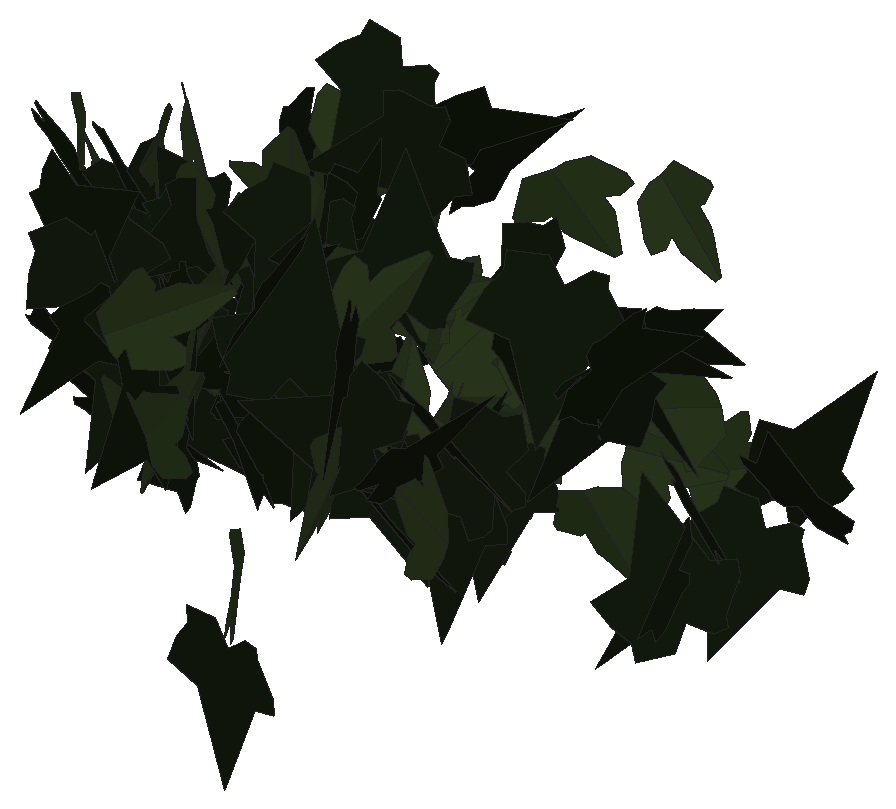
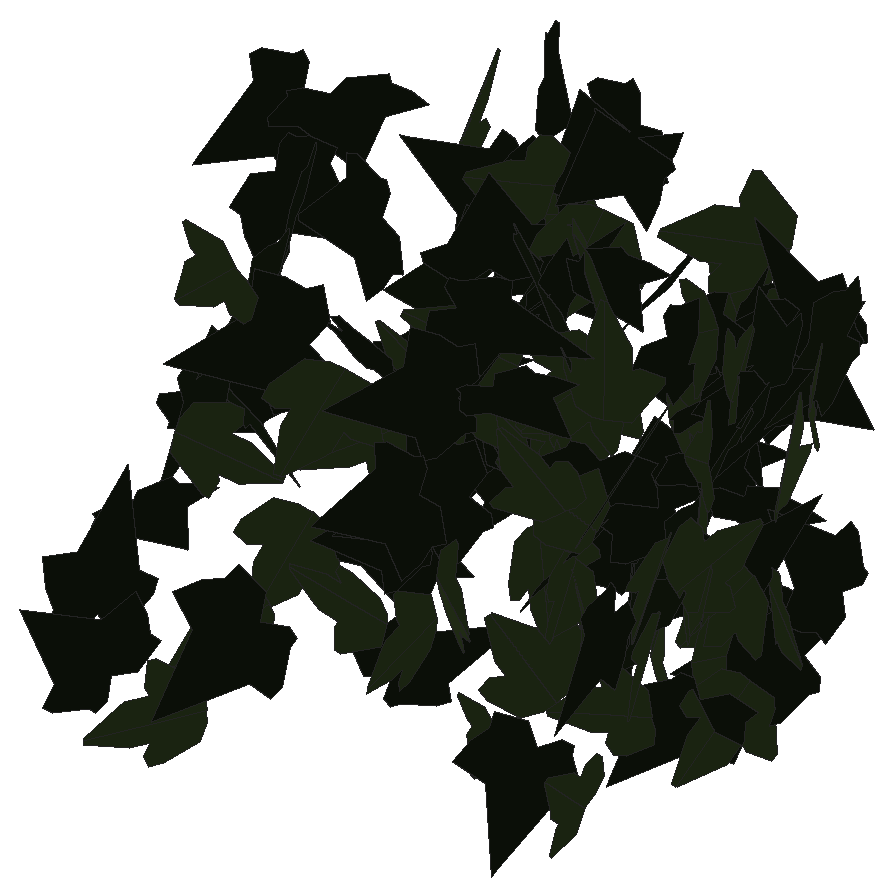
# SketchUp Ruby script. Lengths in inches.
U = 1.inch
M = Sketchup.active_model
def pt(a) = Geom::Point3d.new(a.map { |v| v * U })
def face(e, loops, mat)
  f = e.add_face(loops[0].map { |a| pt(a) })
  loops[1..].each { |l| e.add_face(l.map { |a| pt(a) }).erase! }
  f.material = f.back_material = mat if mat
  f
end
# faces: each face lists its corners as indices into pts; further lists are holes
def faces(e, pts, list, mat = nil) = list.each { |f| face(e, (f[0].is_a?(Array) ? f : [f]).map { |l| l.map { |i| pts[i] } }, mat) }
# xy, xz, yz: faces in a plane at the given z, y or x. An outline is a flat list of corners, or four numbers for a rectangle; further outlines are holes
def ring(l) = l.size == 4 ? [[l[0], l[1]], [l[2], l[1]], [l[2], l[3]], [l[0], l[3]]] : l.each_slice(2).to_a
def flat(e, list, mat, &to3) = list.each { |f| face(e, (f[0].is_a?(Array) ? f : [f]).map { |l| ring(l).map { |u, v| to3.(u, v) } }, mat) }
def xy(e, z, list, mat = nil) = flat(e, list, mat) { |x, y| [x, y, z] }
def xz(e, y, list, mat = nil) = flat(e, list, mat) { |x, z| [x, y, z] }
def yz(e, x, list, mat = nil) = flat(e, list, mat) { |y, z| [x, y, z] }
def lines(e, pts, list) = list.each { |a, b| e.add_line(pt(pts[a]), pt(pts[b])) }
# prism: a flat outline (further loops are holes) pulled along v
def prism(e, loops, v, mat = nil)
  f = face(e, loops, mat); d = Geom::Vector3d.new(v.map { |x| x * U })
  f.pushpull(f.normal.samedirection?(d) ? d.length : -d.length)
end
def box(e, o, s, mat = nil) = prism(e, [[o, [o[0] + s[0], o[1], o[2]], [o[0] + s[0], o[1] + s[1], o[2]], [o[0], o[1] + s[1], o[2]]]], [0, 0, s[2]], mat)
def at(x, y, z, deg = 0) = Geom::Transformation.translation(pt([x, y, z])) * Geom::Transformation.rotation(ORIGIN, Z_AXIS, deg.degrees)
def axes(o, x, y, z) = Geom::Transformation.new([*x, 0, *y, 0, *z, 0, *pt(o).to_a, 1])
def part(name) = M.definitions.add(name)
# library, detail: a bought-in or finely detailed component or shape, given as its bounding box
def library(name, o, s) = part(name).tap { |d| box(d.entities, o, s) }
def detail(e, o, s) = box(e.add_group.entities, o, s)
def put(e, d, t, mat = nil) = e.add_instance(d, t).tap { |i| i.material = mat if mat }
def group(e, t, mat = nil) = e.add_group.tap { |g| g.transformation = t; g.material = mat if mat }.entities
root = M.entities
M.materials.add("efeu1").color = [18, 25, 13]
M.materials.add("efeu2").color = [43, 57, 29]
c1 = part("ivyleaf_10")
p = [[0,0.5,-0.03],[-0.0625,2.02,-0.43],[-0.19,2.01,-0.46],[-0.54,1.05,-0.29],[-0.52,0.625,-0.18],[-0.83,0.76,-0.28],
  [-1.16,0.64,-0.33],[-1.15,0.33,-0.24],[-0.77,-0.39,0.02],[-0.3,-0.51,0.16],[0.04,-0.48,0.23],[-0.02,2.01,-0.4375],
  [-0.06,2.01,-0.43],[0.04,-0.49,0.23],[0.67,-0.49,0.14],[1.38,0.36,-0.2],[1.375,0.51,-0.24],[0.81,0.65,-0.19],
  [0.62,0.59,-0.15],[0.6,1.09,-0.28],[0.5,1.23,-0.31]]
faces(c1.entities,p,[[0,1,2,3,4,5,6,7,8,9,10],[11,12,0,13,14,15,16,17,18,19,20]],"efeu2")
c2 = part("ivyleaf_9")
p = [[1.54,2.16,1.25],[1.36,2.04,1.19],[-0.21,0.99,0.68],[-0.71,1.11,0.82],[-0.85,0.86,0.67],[-0.8,0.17,0.21],
  [-0.9,-0.01,0.1],[-0.67,-0.16,-0.02],[-0.08,-0.08,-0.05],[-0.03,-0.6,-0.4],[0.65,-0.88,-0.66],[0.83,-0.6,-0.49],
  [1.29,-0.42,-0.43],[1.8125,-0.07,-0.26],[1.21,0.44,0.15]]
faces(c2.entities,p,[[0,1,2,3,4,5,6,7,8,9,10,11,12,13,14]],"efeu1")
put(root,c1,axes([545.16,132.69,171.34],[0.0468,-0.12777,0.80813],[0.64002,-0.49853,-0.11589],[0.50968,0.63775,0.07132]))
put(root,c2,axes([545.81,137.93,168.91],[0.10586,0.00489,-0.89003],[-0.6226,0.64092,-0.07053],[0.63604,0.62656,0.07909]))
put(root,c1,axes([545.47,133.17,169.69],[-0.56596,0.35181,0.69168],[0.48132,-0.51238,0.65445],[0.60871,0.73226,0.12562]))
put(root,c2,axes([545.18,131.93,167.14],[0.64135,0.09368,-0.50962],[0.50203,0.08838,0.64805],[0.12825,-0.81439,0.01171]))
put(root,c1,axes([546.17,135.08,168.43],[-0.26299,-0.24108,-0.73681],[-0.41993,-0.60973,0.34938],[-0.65167,0.4902,0.07221]))
put(root,c1,axes([546.54,132.27,166.55],[-0.20531,0.1267,0.79196],[-0.75894,0.23367,-0.23413],[-0.25936,-0.78406,0.0582]))
put(root,c1,axes([546.12,136.41,167.81],[-0.37564,0.62219,0.36467],[-0.21105,0.29833,-0.72641],[-0.68961,-0.43022,0.02367]))
put(root,c2,axes([545.58,131.3,172.08],[0.90183,-0.44317,-0.15553],[-0.13097,0.08607,-1.00465],[0.45103,0.91108,0.01925]))
put(root,c1,axes([546.14,133.78,165.17],[-0.40054,-0.55747,-0.63228],[0.33936,0.53415,-0.68593],[0.77161,-0.5243,-0.02654]))
put(root,c2,axes([545.66,132.53,165.8],[0.77933,-0.17074,0.48973],[0.48275,-0.0843,-0.79762],[0.18957,0.91656,0.01787]))
put(root,c1,axes([545.93,134.91,170.88],[0.18655,-0.26248,0.75231],[0.70853,-0.2988,-0.27994],[0.36448,0.71518,0.15914]))
put(root,c1,axes([546.42,139.27,167.89],[-0.33228,-0.69013,0.41546],[0.17481,0.37693,0.76594],[-0.78634,0.37542,-0.00528]))
put(root,c2,axes([546.96,133.66,166.93],[0.00388,0.08176,1.01596],[-0.82421,-0.59744,0.05123],[0.59962,-0.82174,0.06384]))
put(root,c1,axes([546.66,137.79,164.59],[0.03621,0.51412,-0.64767],[0.0814,0.64293,0.5149],[0.82291,-0.08622,-0.02243]))
put(root,c1,axes([546.3125,133.61,167.44],[-0.74533,0.07894,-0.51976],[0.5144,-0.07659,-0.74928],[-0.10849,-0.90542,0.01806]))
put(root,c1,axes([546.33,134.86,167.47],[-0.43425,0.20169,0.66637],[0.57812,-0.33315,0.47759],[0.38794,0.72224,0.0342]))
put(root,c1,axes([546.875,135.22,168.66],[-0.27817,0.77347,0.24377],[-0.0926,0.22573,-0.8219],[-0.80567,-0.29299,0.0103]))
put(root,c2,axes([546.48,134.53,165.37],[-0.05567,-0.38101,-0.81682],[0.26644,0.77484,-0.37959],[0.86103,-0.2644,0.06465]))
put(root,c2,axes([546.69,132.27,171.05],[0.01681,-0.66358,-0.6588],[-0.00182,0.65889,-0.66371],[0.93507,0.01322,0.01055]))
put(root,c1,axes([546.8,133.1,171.4],[0.05216,-0.14231,-0.80456],[0.16397,-0.78798,0.15001],[-0.80043,-0.1707,-0.0217]))
put(root,c1,axes([546.83,133.8125,165.81],[0.1364,-0.29183,0.87678],[0.4245,-0.76744,-0.32148],[0.82079,0.44541,0.02056]))
put(root,c2,axes([546.61,135.62,167.42],[0.19867,-0.5933,0.60102],[0.2685,-0.54102,-0.62282],[0.80071,0.32862,0.05972]))
put(root,c2,axes([546.55,132.28,171.2],[0.66923,-0.24845,-0.60284],[0.56033,-0.22261,0.71378],[-0.33343,-0.87277,-0.01045]))
put(root,c1,axes([546.86,136.01,165.64],[0.1082,0.05044,0.83793],[0.73557,0.40139,-0.11914],[-0.40448,0.74344,0.00748]))
put(root,c2,axes([547.05,129.99,170.95],[-0.13394,0.09954,0.9014],[0.64776,-0.62719,0.16551],[0.63469,0.66112,0.0213]))
put(root,c2,axes([547.73,131.45,167.94],[-0.72157,-0.40686,-0.14062],[0.12421,0.066,-0.82836],[0.41216,-0.73217,0.00347]))
put(root,c1,axes([547.4,133.38,167.24],[-0.54542,0.41996,0.55461],[0.4431,-0.33359,0.68835],[0.53631,0.70271,-0.00468]))
put(root,c2,axes([547.25,132.66,169.78],[0.13773,-0.58989,0.63667],[0.16032,-0.61626,-0.60565],[0.85301,0.21107,0.01103]))
put(root,c2,axes([547.85,137.7,165.22],[0.50874,0.6559,-0.09298],[-0.06824,-0.06472,-0.82995],[-0.65893,0.5131,0.01417]))
put(root,c2,axes([547.63,133.04,167.75],[0.7859,-0.2609,-0.21098],[-0.19994,0.06735,-0.82808],[0.26945,0.81094,0.0009]))
put(root,c2,axes([548.26,129.63,169.88],[-0.1336,0.27227,-0.80449],[0.18616,-0.78519,-0.29666],[-0.82866,-0.22029,0.06306]))
put(root,c2,axes([548.13,132.27,170.29],[-0.31648,-0.66548,0.32812],[-0.11479,-0.30851,-0.73643],[0.73304,-0.33562,0.02634]))
put(root,c2,axes([547.8125,129.76,171.14],[-0.14827,-0.74749,-0.57441],[0.21913,0.53822,-0.75695],[0.91688,-0.24951,0.08802]))
put(root,c2,axes([548.05,132.17,165.77],[-0.07961,-0.30213,0.75968],[-0.09596,-0.75454,-0.31014],[0.8119,-0.1188,0.03783]))
put(root,c2,axes([548.39,131.83,168.8],[-0.48632,-0.72464,-0.09334],[0.05059,0.07845,-0.8727],[0.72887,-0.48894,-0.0017]))
put(root,c1,axes([548.1,136.88,170.27],[0.66083,0.15914,-0.47947],[0.46747,0.10672,0.67971],[0.19156,-0.80945,-0.00465]))
put(root,c2,axes([549.04,133.41,165.19],[0.13334,-0.42054,0.73686],[-0.07845,0.7366,0.43459],[-0.84479,-0.13478,0.07595]))
put(root,c2,axes([549.04,132.07,171.22],[-0.05277,-0.10494,-0.85907],[0.07109,-0.85828,0.10048],[-0.86253,-0.06432,0.06084]))
put(root,c2,axes([548.43,131.22,169.7],[-0.45887,-0.06523,-0.85105],[0.83339,0.17448,-0.46272],[0.18438,-0.951,-0.02653]))
put(root,c1,axes([548.46,131.86,171.5],[-0.37592,0.35119,-0.72693],[0.53616,-0.49089,-0.51442],[-0.60357,-0.6548,-0.00422]))
put(root,c1,axes([548.8,139.1,168.99],[0.47252,-0.57439,0.48351],[0.30055,-0.37881,-0.74374],[0.68802,0.55996,-0.00717]))
put(root,c2,axes([549.29,134.09,168.18],[0.09813,-0.90153,0.2624],[-0.01305,0.26249,0.90673],[-0.93885,-0.09788,0.01482]))
put(root,c1,axes([549.17,133.9,170.77],[-0.85642,-0.13948,0.0913],[0.09084,0.01019,0.86769],[-0.13977,0.86121,0.00452]))
put(root,c2,axes([549.33,136.95,172.19],[-0.63275,-0.55748,0.05586],[-0.03963,-0.03952,-0.84329],[0.55887,-0.63398,0.00344]))
put(root,c1,axes([549.23,131.6,169.74],[0.28382,-0.62548,0.57367],[0.26298,-0.51032,-0.68651],[0.80695,0.38631,0.02196]))
put(root,c1,axes([549.65,130.17,168.34],[0.19399,-0.80251,0.49862],[0.11645,-0.48483,-0.82562],[0.93759,0.22626,-0.00062]))
put(root,c2,axes([549.18,132.03,167.55],[0.22559,0.04435,0.93346],[0.85859,0.3693,-0.22504],[-0.36897,0.88648,0.04705]))
put(root,c2,axes([549.42,133.8,169.15],[-0.25371,-0.54509,-0.63173],[0.32089,0.54577,-0.59979],[0.77022,-0.40693,0.04179]))
put(root,c1,axes([550.23,133.3125,165.36],[0.37328,-0.29831,0.723],[-0.58107,0.43047,0.47761],[-0.52353,-0.69048,-0.0146]))
put(root,c1,axes([549.53,136.74,164.51],[0.6512,-0.03728,0.52916],[0.52602,-0.06297,-0.65177],[0.0686,0.83673,-0.02548]))
put(root,c1,axes([550.09,133.74,166.36],[-0.01477,-0.60436,-0.67066],[0.0078,0.67064,-0.60452],[0.90276,-0.01568,-0.00575]))
put(root,c2,axes([549.74,131.86,166.56],[0.14508,-0.47662,0.66592],[0.23324,-0.62423,-0.49759],[0.78499,0.27356,0.02478]))
put(root,c1,axes([549.82,131.52,164.05],[0.11579,-0.11647,0.92285],[0.69576,-0.60639,-0.16383],[0.61736,0.70524,0.01155]))
put(root,c1,axes([549.88,133.43,170.73],[-0.79224,0.07311,-0.67145],[0.6691,-0.05628,-0.79559],[-0.09217,-1.03697,-0.00415]))
put(root,c1,axes([549.74,134.01,168.02],[-0.34919,-0.15127,0.8439],[0.79527,0.28326,0.37984],[-0.32029,0.86825,0.0231]))
put(root,c2,axes([550.41,138.07,169.97],[-0.1339,0.58279,-0.65196],[-0.19338,0.6235,0.59706],[0.85282,0.23288,0.03302]))
put(root,c2,axes([550.26,128.59,169.34],[0.19336,-0.32379,-0.95206],[0.64646,-0.70261,0.37024],[-0.7703,-0.67093,0.07174]))
put(root,c2,axes([550.27,133.86,166.68],[0.02412,-0.82645,0.28701],[0.02709,-0.28627,-0.82662],[0.87445,0.03167,0.01769]))
put(root,c1,axes([550.68,133.9,166.92],[-0.13182,-0.91856,-0.06434],[0.01188,0.06329,-0.92796],[0.92073,-0.13232,0.00277]))
put(root,c1,axes([550.25,127.875,170.97],[-0.08395,-0.32421,0.94485],[0.37171,0.86995,0.33153],[-0.92719,0.37812,0.04736]))
put(root,c2,axes([550.1875,131.99,166.06],[0.01643,-0.08115,0.8107],[0.74082,-0.33604,-0.04865],[0.33914,0.73796,0.067]))
put(root,c1,axes([550.85,131.94,169.36],[-0.36836,-0.58269,-0.4797],[0.30729,0.37175,-0.68754],[0.68936,-0.47708,0.05015]))
put(root,c1,axes([550.65,127.78,168.83],[-0.76693,-0.06032,0.58543],[0.5859,0.01263,0.76884],[-0.05562,0.96475,0.02654]))
put(root,c2,axes([551.68,135.07,172.21],[-0.17002,-0.2,-0.85981],[-0.51169,-0.69118,0.26195],[-0.71934,0.53893,0.01688]))
put(root,c2,axes([550.61,136.68,171.42],[0.47077,0.18764,0.67897],[0.6068,0.30675,-0.50551],[-0.35778,0.76716,0.03606]))
put(root,c2,axes([551.21,132.02,172.03],[-0.68965,-0.57396,-0.11611],[0.0952,0.06711,-0.89719],[0.57779,-0.69613,0.00925]))
put(root,c2,axes([551.8,132.42,171.47],[-0.22942,0.59231,0.8468],[-0.32445,0.78226,-0.63507],[-0.98113,-0.39719,0.012]))
put(root,c1,axes([550.73,132.86,169.37],[0.66572,0.15294,0.54034],[0.51472,0.1689,-0.68197],[-0.22454,0.84061,0.03871]))
put(root,c1,axes([551.28,131.89,172.11],[0.70973,-0.65256,-0.03151],[-0.02183,0.02281,-0.96413],[0.65295,0.71007,0.00202]))
put(root,c1,axes([550.9,132.36,168.94],[0.25032,0.20234,-0.90415],[0.69152,0.58252,0.32181],[0.61663,-0.73541,0.00614]))
put(root,c2,axes([551.69,132.625,171.15],[-0.1147,-0.20503,0.845],[-0.38448,-0.75251,-0.23477],[0.77989,-0.40114,0.00853]))
put(root,c2,axes([551.3,135.51,168.51],[0.70923,0.1518,0.48928],[0.47792,0.10484,-0.72529],[-0.18448,0.85523,0.00207]))
put(root,c1,axes([552.17,135.73,165.42],[-0.01734,0.16119,0.86373],[-0.26542,0.82258,-0.15884],[-0.83759,-0.264,0.03245]))
put(root,c2,axes([551.85,133.63,170.91],[0.34291,-0.85103,-0.29467],[-0.07748,0.28626,-0.91691],[0.89726,0.34997,0.03343]))
put(root,c2,axes([552.79,135.65,164.25],[-0.14715,-0.04072,0.84102],[-0.80343,-0.24865,-0.15261],[0.25192,-0.81678,0.00453]))
put(root,c1,axes([552.24,130.46,171.59],[-0.50314,-0.67439,-0.51289],[0.30219,0.41444,-0.84138],[0.79155,-0.58689,-0.0048]))
put(root,c2,axes([552.17,135.83,167.64],[0.68307,-0.26172,0.43688],[0.40721,-0.15828,-0.73149],[0.30586,0.79523,-0.0018]))
put(root,c2,axes([553.19,127.96,172.4375],[-0.32042,0.46666,-0.8797],[-0.4941,0.72783,0.56607],[0.86459,0.58889,-0.00252]))
put(root,c1,axes([552.45,133.1,170.15],[-0.27836,-0.18189,0.85888],[0.69605,0.50339,0.3322],[-0.53504,0.7495,-0.01467]))
put(root,c1,axes([553.07,137.26,170.94],[-0.72191,-0.43332,-0.42296],[0.37441,0.19783,-0.84172],[0.4759,-0.81296,0.02062]))
put(root,c1,axes([553.18,132.19,167.78],[0.9478,-0.12497,0.0511],[-0.04734,0.03178,0.95567],[-0.12644,-0.94864,0.02528]))
put(root,c1,axes([553.47,133.47,168.18],[0.40855,-0.74823,-0.27185],[-0.10636,0.25151,-0.85211],[0.78895,0.42137,0.0259]))
put(root,c1,axes([553.2,133.62,169.74],[-0.00746,-0.2389,-0.91823],[0.38449,0.83872,-0.22134],[0.8674,-0.37384,0.09021]))
put(root,c1,axes([552.75,136.65,166.01],[0.20567,-0.11772,-0.82357],[0.81726,-0.1301,0.22269],[-0.15561,-0.83884,0.08104]))
put(root,c2,axes([553.1875,139.37,166.82],[0.63727,0.57336,0.31985],[0.2324,0.21988,-0.85721],[-0.61403,0.67829,0.00751]))
put(root,c2,axes([553.67,131.71,171.01],[-0.7418,-0.40603,0.51882],[0.46449,0.23175,0.84549],[-0.46721,0.87506,0.01682]))
put(root,c1,axes([553.57,133.47,168.17],[-0.16153,-0.45799,-0.75211],[0.27817,0.69897,-0.48537],[0.83549,-0.32126,0.01619]))
put(root,c2,axes([553.64,134.74,166.32],[-0.628,-0.55094,-0.35137],[0.25787,0.23883,-0.83537],[0.60042,-0.67882,-0.00874]))
put(root,c2,axes([553.8125,128.14,171.21],[-0.70632,-0.31356,0.62057],[0.56165,0.26414,0.77272],[-0.40985,0.90234,-0.01055]))
put(root,c2,axes([553.51,131.49,167.67],[-0.16171,-0.63797,-0.51265],[0.13331,0.49505,-0.65811],[0.80749,-0.20949,0.00598]))
put(root,c2,axes([553.89,129.99,170.19],[-0.60527,-0.76493,0.00311],[-0.00158,-0.00272,-0.97543],[0.76493,-0.60527,0.00045]))
put(root,c2,axes([553.17,131.375,166.61],[0.52185,-0.47308,0.56669],[0.44806,-0.34856,-0.70359],[0.58668,0.68701,0.03326]))
put(root,c2,axes([554.53,134.86,170.52],[-0.87131,0.21897,0.14719],[-0.14336,0.03346,-0.8984],[-0.2215,-0.88302,0.00245]))
put(root,c1,axes([553.5,133.42,169.1],[0.7129,-0.10552,-0.53238],[0.54202,0.09334,0.70731],[-0.02784,-0.88484,0.1381]))
put(root,c2,axes([553.65,131.21,168.91],[0.17319,-0.53157,0.6471],[0.22488,-0.607,-0.55881],[0.80668,0.28334,0.01686]))
put(root,c1,axes([553.76,134.92,168.78],[0.35573,0.29059,0.78873],[0.63634,0.46647,-0.45887],[-0.54918,0.72873,-0.02079]))
put(root,c1,axes([554.14,129.68,171.65],[0.15937,0.34549,-0.88816],[0.38759,0.79915,0.38041],[0.87061,-0.41902,-0.00678]))
put(root,c2,axes([554.94,132.04,168.21],[-0.2914,0.81658,0.2578],[-0.09475,0.2399,-0.86698],[-0.85105,-0.30631,0.00825]))
put(root,c2,axes([555.62,128.2,170.2],[-0.19864,0.01983,0.8844],[-0.84493,-0.27271,-0.18366],[0.262,-0.86443,0.07823]))
put(root,c2,axes([554.96,131.7,167.45],[-0.72751,-0.27777,-0.57547],[0.52874,0.22803,-0.77848],[0.35884,-0.89913,-0.01965]))
put(root,c1,axes([554.83,137.5625,165.63],[0.08556,0.35048,0.7985],[0.18576,0.7766,-0.36077],[-0.85202,0.20451,0.00153]))
put(root,c1,axes([554.83,139.56,164.39],[0.01669,0.07725,0.92151],[0.33051,0.86028,-0.0781],[-0.86366,0.33071,-0.01208]))
put(root,c2,axes([555.76,131.95,168.07],[-0.48516,-0.24244,0.72749],[-0.65445,-0.31773,-0.54234],[0.39963,-0.81466,-0.00498]))
put(root,c2,axes([555.0625,124.6875,167.12],[0.104,-0.92787,0.30072],[0.05473,-0.29639,-0.93345],[0.97384,0.11575,0.02035]))
put(root,c1,axes([555.19,127.73,169.78],[0.1796,-0.37409,0.90819],[0.4549,-0.78658,-0.41396],[0.87053,0.48821,0.02895]))
put(root,c2,axes([554.94,130.53,169.7],[0.68924,-0.47271,0.40824],[0.33898,-0.22753,-0.83576],[0.52461,0.76808,0.00367]))
put(root,c2,axes([555.4,127.9,172.6875],[-0.24287,0.12383,-0.9645],[0.85338,-0.44946,-0.27259],[-0.46619,-0.88726,0.00348]))
put(root,c1,axes([555.7,134.95,165.96],[-0.8588,-0.09893,-0.32733],[0.32491,0.03983,-0.86448],[0.10662,-0.9182,-0.00224]))
put(root,c1,axes([557.08,136.18,168.03],[0.25255,0.01161,-0.84553],[-0.84558,0.01163,-0.25241],[0.00783,0.88237,0.01445]))
put(root,c2,axes([556.19,127.99,169.78],[0.17993,0.8728,-0.18622],[0.01892,0.18619,0.89095],[0.89224,-0.17996,0.01866]))
put(root,c2,axes([555.87,134.6,169.8],[0.70266,0.06434,0.59038],[0.58974,0.03219,-0.70541],[-0.06999,0.91719,-0.01665]))
put(root,c1,axes([556.15,136.52,172.07],[0.54723,0.0551,0.68695],[0.68143,0.08767,-0.54987],[-0.10286,0.87388,0.01185]))
put(root,c2,axes([556.6,139.51,164.66],[-0.20043,-0.14482,0.9022],[0.74153,0.51393,0.24723],[-0.53392,0.76812,0.00468]))
put(root,c2,axes([556.23,131.87,171.17],[0.13502,-0.0047,-0.9318],[0.89417,0.26557,0.12823],[0.26218,-0.90331,0.04255]))
put(root,c2,axes([557.34,133.67,170.2],[0.76406,-0.44787,-0.24673],[-0.2026,0.14215,-0.88544],[0.46948,0.79023,0.01944]))
put(root,c2,axes([557.69,138.4375,165.2],[0.83969,-0.32422,0.23219],[-0.21625,0.08454,0.90011],[-0.33506,-0.86709,0.00094]))
put(root,c2,axes([557.3,133.03,171.3125],[0.30454,-0.14624,-0.91366],[0.82104,-0.40083,0.33783],[-0.42667,-0.8757,-0.00205]))
put(root,c2,axes([557.83,131.23,172.95],[-0.51822,-0.83814,-0.24813],[0.14411,0.20259,-0.98528],[0.86213,-0.53766,0.01554]))
put(root,c1,axes([558.15,126.97,169.78],[-0.41864,0.68437,0.57434],[0.25854,-0.51433,0.80132],[0.85521,0.4905,0.0389]))
put(root,c2,axes([558.8,131.63,171.1],[-0.08823,0.2841,-0.87622],[0.23648,-0.84375,-0.29738],[-0.89026,-0.25228,0.00785]))
put(root,c2,axes([558.72,136.07,165.98],[-0.44718,-0.7709,0.06351],[-0.03208,-0.05481,-0.89121],[0.77285,-0.44833,-0.00024]))
put(root,c2,axes([558.625,133.76,167.9],[0.76016,-0.16583,-0.50191],[-0.47519,0.17069,-0.77609],[0.23153,0.89478,0.05503]))
put(root,c2,axes([559.53,132.47,166.99],[-0.80448,0.41023,-0.20214],[0.17425,-0.10322,-0.90295],[-0.42283,-0.82304,0.01249]))
put(root,c2,axes([559.64,132.57,166.05],[-0.76374,-0.52119,0.25655],[0.22287,0.12845,0.92444],[-0.53646,0.79537,0.01882]))
put(root,c2,axes([559.26,130.47,172.125],[-0.10249,0.40331,-0.86016],[-0.29443,0.80906,0.41444],[0.90324,0.3095,0.03749]))
